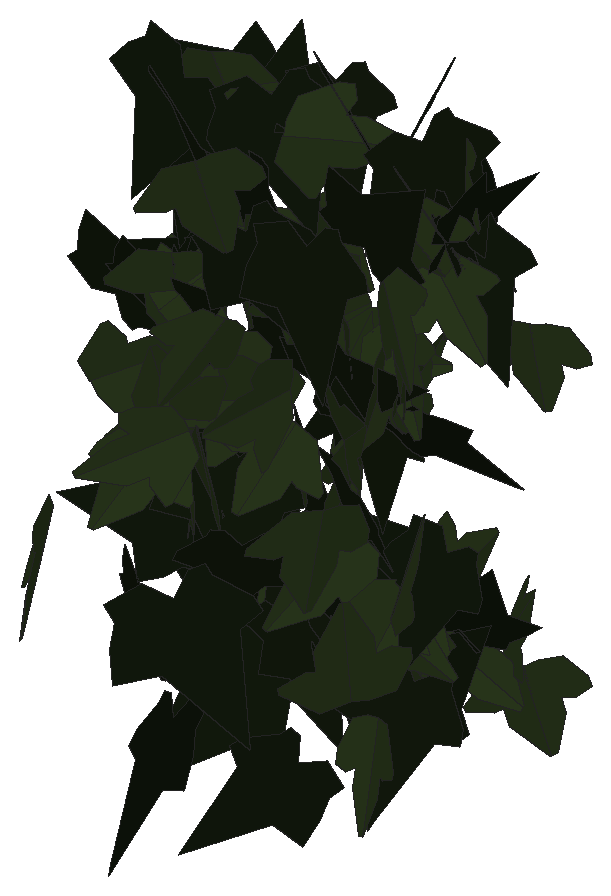
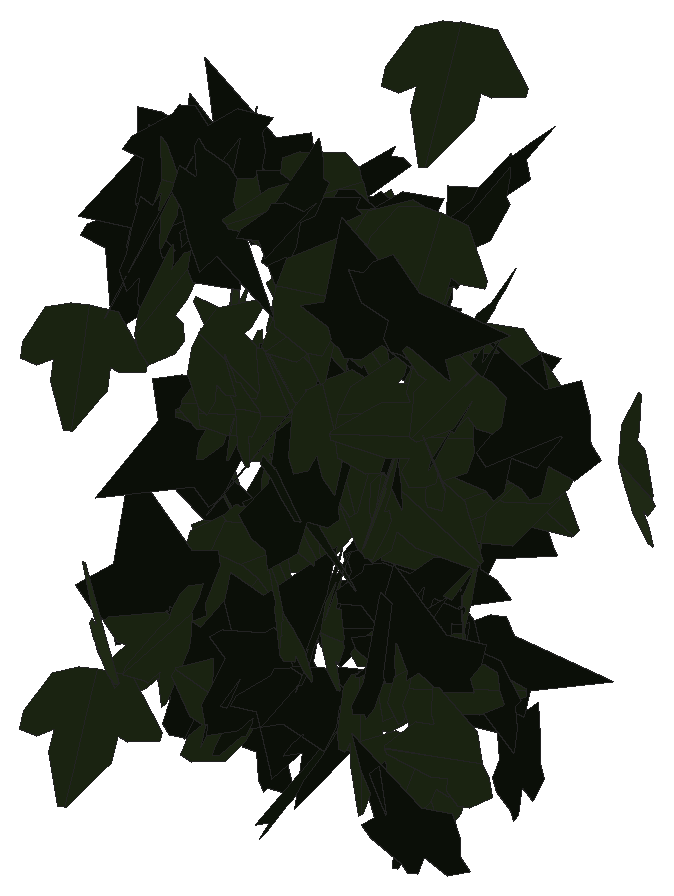
# SketchUp Ruby script. Lengths in inches.
U = 1.inch
M = Sketchup.active_model
def pt(a) = Geom::Point3d.new(a.map { |v| v * U })
def face(e, loops, mat)
  f = e.add_face(loops[0].map { |a| pt(a) })
  loops[1..].each { |l| e.add_face(l.map { |a| pt(a) }).erase! }
  f.material = f.back_material = mat if mat
  f
end
# faces: each face lists its corners as indices into pts; further lists are holes
def faces(e, pts, list, mat = nil) = list.each { |f| face(e, (f[0].is_a?(Array) ? f : [f]).map { |l| l.map { |i| pts[i] } }, mat) }
# xy, xz, yz: faces in a plane at the given z, y or x. An outline is a flat list of corners, or four numbers for a rectangle; further outlines are holes
def ring(l) = l.size == 4 ? [[l[0], l[1]], [l[2], l[1]], [l[2], l[3]], [l[0], l[3]]] : l.each_slice(2).to_a
def flat(e, list, mat, &to3) = list.each { |f| face(e, (f[0].is_a?(Array) ? f : [f]).map { |l| ring(l).map { |u, v| to3.(u, v) } }, mat) }
def xy(e, z, list, mat = nil) = flat(e, list, mat) { |x, y| [x, y, z] }
def xz(e, y, list, mat = nil) = flat(e, list, mat) { |x, z| [x, y, z] }
def yz(e, x, list, mat = nil) = flat(e, list, mat) { |y, z| [x, y, z] }
def lines(e, pts, list) = list.each { |a, b| e.add_line(pt(pts[a]), pt(pts[b])) }
# prism: a flat outline (further loops are holes) pulled along v
def prism(e, loops, v, mat = nil)
  f = face(e, loops, mat); d = Geom::Vector3d.new(v.map { |x| x * U })
  f.pushpull(f.normal.samedirection?(d) ? d.length : -d.length)
end
def box(e, o, s, mat = nil) = prism(e, [[o, [o[0] + s[0], o[1], o[2]], [o[0] + s[0], o[1] + s[1], o[2]], [o[0], o[1] + s[1], o[2]]]], [0, 0, s[2]], mat)
def at(x, y, z, deg = 0) = Geom::Transformation.translation(pt([x, y, z])) * Geom::Transformation.rotation(ORIGIN, Z_AXIS, deg.degrees)
def axes(o, x, y, z) = Geom::Transformation.new([*x, 0, *y, 0, *z, 0, *pt(o).to_a, 1])
def part(name) = M.definitions.add(name)
# library, detail: a bought-in or finely detailed component or shape, given as its bounding box
def library(name, o, s) = part(name).tap { |d| box(d.entities, o, s) }
def detail(e, o, s) = box(e.add_group.entities, o, s)
def put(e, d, t, mat = nil) = e.add_instance(d, t).tap { |i| i.material = mat if mat }
def group(e, t, mat = nil) = e.add_group.tap { |g| g.transformation = t; g.material = mat if mat }.entities
root = M.entities
M.materials.add("efeu1").color = [18, 25, 13]
M.materials.add("efeu2").color = [43, 57, 29]
c1 = part("ivyleaf_10")
p = [[0,0.5,-0.03],[-0.0625,2.02,-0.43],[-0.19,2.01,-0.46],[-0.54,1.05,-0.29],[-0.52,0.625,-0.18],[-0.83,0.76,-0.28],
  [-1.16,0.64,-0.33],[-1.15,0.33,-0.24],[-0.77,-0.39,0.02],[-0.3,-0.51,0.16],[0.04,-0.48,0.23],[-0.02,2.01,-0.4375],
  [-0.06,2.01,-0.43],[0.04,-0.49,0.23],[0.67,-0.49,0.14],[1.38,0.36,-0.2],[1.375,0.51,-0.24],[0.81,0.65,-0.19],
  [0.62,0.59,-0.15],[0.6,1.09,-0.28],[0.5,1.23,-0.31]]
faces(c1.entities,p,[[0,1,2,3,4,5,6,7,8,9,10],[11,12,0,13,14,15,16,17,18,19,20]],"efeu2")
c2 = part("ivyleaf_9")
p = [[1.54,2.16,1.25],[1.36,2.04,1.19],[-0.21,0.99,0.68],[-0.71,1.11,0.82],[-0.85,0.86,0.67],[-0.8,0.17,0.21],
  [-0.9,-0.01,0.1],[-0.67,-0.16,-0.02],[-0.08,-0.08,-0.05],[-0.03,-0.6,-0.4],[0.65,-0.88,-0.66],[0.83,-0.6,-0.49],
  [1.29,-0.42,-0.43],[1.8125,-0.07,-0.26],[1.21,0.44,0.15]]
faces(c2.entities,p,[[0,1,2,3,4,5,6,7,8,9,10,11,12,13,14]],"efeu1")
put(root,c1,axes([537.25,133.6,181.46],[0.57557,0.24818,0.51363],[0.45043,0.25001,-0.62555],[-0.35004,0.72979,0.03962]))
put(root,c1,axes([537.01,133.92,174.57],[0.1954,0.05851,0.86892],[0.85639,0.14889,-0.20261],[-0.15823,0.87809,-0.02355]))
put(root,c2,axes([537.17,131.61,179.2],[-0.21585,-0.03871,0.90493],[0.74592,-0.53531,0.15502],[0.5138,0.76087,0.1551]))
put(root,c2,axes([538.46,134.02,182.43],[-0.26612,0.12962,0.83782],[-0.7365,0.39956,-0.29576],[-0.41988,-0.78301,-0.01223]))
put(root,c2,axes([538.63,131.59,174.97],[-0.37083,-0.27346,-0.68713],[-0.49143,-0.4833,0.45756],[-0.55265,0.61326,0.05419]))
put(root,c2,axes([537.68,133.11,181.74],[0.09063,-0.70819,0.53318],[0.07182,-0.52833,-0.71396],[0.88355,0.11558,0.00334]))
put(root,c2,axes([537.77,133.33,180.37],[-0.06348,-0.47882,0.77083],[0.07599,-0.7728,-0.47379],[0.90425,0.03133,0.09392]))
put(root,c1,axes([538.62,132.86,174.82],[-0.01712,-0.07094,0.79621],[-0.34555,-0.71749,-0.07135],[0.72082,-0.34564,-0.0153]))
put(root,c1,axes([538.375,133.14,183.65],[-0.81606,-0.18859,-0.13277],[0.12874,0.03255,-0.83757],[0.19136,-0.82615,-0.00269]))
put(root,c2,axes([537.98,131.24,172.64],[-0.04193,-0.01194,0.86813],[0.34833,-0.79636,0.00587],[0.79527,0.34817,0.0432]))
put(root,c1,axes([538.08,130.35,178.27],[-0.26014,-0.32007,0.79563],[0.51114,0.60975,0.41242],[-0.68863,0.57351,0.00556]))
put(root,c1,axes([538.09,133.42,179.41],[0.1015,-0.19936,-0.74319],[0.47513,-0.57341,0.21871],[-0.60525,-0.48357,0.04705]))
put(root,c1,axes([537.95,133.3,180.11],[0.02509,-0.0054,0.92465],[0.67,0.63759,-0.01446],[-0.63726,0.67014,0.0212]))
put(root,c2,axes([538.37,131.97,183.875],[-0.15974,-0.84049,0.4832],[-0.04558,-0.48266,-0.85462],[0.96841,-0.16136,0.03948]))
put(root,c2,axes([538.29,133.49,172.17],[-0.40577,0.25126,0.66866],[0.55816,-0.36837,0.47713],[0.44575,0.68998,0.01123]))
put(root,c2,axes([538.6,133.19,175.41],[-0.64239,-0.06086,0.45253],[0.45611,-0.12191,0.63107],[0.02126,0.77626,0.13459]))
put(root,c2,axes([537.97,131.61,179.07],[-0.02434,-0.21976,0.96131],[0.74537,-0.63368,-0.12599],[0.64562,0.7233,0.1817]))
put(root,c2,axes([538.12,132.31,183.25],[0.20488,-0.61087,0.62806],[0.27591,-0.5672,-0.64168],[0.83156,0.3387,0.05817]))
put(root,c1,axes([538.49,134.51,178.64],[-0.32078,0.40567,0.5683],[0.32601,-0.46603,0.51669],[0.61745,0.45681,0.02243]))
put(root,c1,axes([538.86,131.2,180.4],[-0.86672,-0.50452,-0.01723],[0.01642,0.00604,-1.00286],[0.50454,-0.86687,0.00304]))
put(root,c1,axes([538.48,133.28,173.79],[0.66238,0.43416,0.28408],[0.2397,0.15251,-0.79197],[-0.46015,0.7044,-0.00362]))
put(root,c1,axes([538.92,131.05,177.34],[-0.49938,-0.75998,-0.32042],[-0.17716,-0.26699,0.90937],[-0.80551,0.52987,-0.00136]))
put(root,c2,axes([538.4,131.82,175.14],[-0.31705,-0.13686,-0.90242],[0.87432,0.22871,-0.34187],[0.26202,-0.92875,0.04879]))
put(root,c1,axes([538.88,133.23,175.34],[-0.00253,0.18198,-0.75905],[-0.07402,-0.75569,-0.18093],[-0.77704,0.07139,0.01971]))
put(root,c1,axes([538.6,131.88,175.71],[-0.05133,-0.08634,0.89803],[0.72856,-0.53447,-0.00975],[0.53209,0.72349,0.09998]))
put(root,c2,axes([539.05,133.6,181.67],[-0.76145,-0.03775,0.58295],[0.58283,-0.11392,0.75392],[0.03954,0.95219,0.11331]))
put(root,c2,axes([539.24,133.28,175.1],[-0.11503,-0.49954,0.70126],[0.23468,0.66251,0.51043],[-0.82839,0.25706,0.04723]))
put(root,c1,axes([538.77,127.33,176.54],[0.4502,-0.49021,0.75163],[0.50259,-0.55892,-0.66555],[0.74341,0.67472,-0.00523]))
put(root,c1,axes([539.34,129.83,177.33],[0.52573,0.45595,-0.51321],[-0.38248,-0.34225,-0.69588],[-0.57008,0.65011,-0.00641]))
put(root,c1,axes([538.96,132.59,180.57],[-0.49848,0.52672,-0.46065],[0.30608,-0.34447,-0.7251],[-0.62924,-0.58483,0.01221]))
put(root,c1,axes([539.73,132.21,177.46],[-0.15474,-0.11552,-0.93869],[-0.73583,-0.58286,0.19303],[-0.59417,0.7519,0.00542]))
put(root,c1,axes([538.79,132.37,172.22],[-0.48485,-0.00356,0.85233],[0.79903,-0.34323,0.4531],[0.29669,0.91855,0.17261]))
put(root,c1,axes([538.85,131.23,179.86],[0.57569,0.06226,-0.5923],[0.5811,0.12173,0.5776],[0.13046,-0.81696,0.04092]))
put(root,c1,axes([539.87,132.4,178.15],[-0.49317,-0.46191,0.76436],[-0.51842,-0.56293,-0.67467],[0.72722,-0.71455,0.0374]))
put(root,c1,axes([539.53,133.23,183.08],[-0.11115,-0.46317,0.65253],[-0.1139,-0.64293,-0.47576],[0.79206,-0.15745,0.02316]))
put(root,c2,axes([539.49,132.09,172.17],[-0.02978,-0.08491,0.96584],[0.22835,0.9385,0.08955],[-0.94229,0.23012,-0.00882]))
put(root,c1,axes([539.8125,129.71,177.78],[0.22347,0.19537,-0.81594],[-0.65316,-0.48946,-0.29609],[-0.5266,0.69001,0.021]))
put(root,c1,axes([539.5,133.54,180.03],[-0.17061,-0.18924,0.88257],[0.04144,-0.89889,-0.18472],[0.90168,0.00551,0.17548]))
put(root,c1,axes([539.7,131.17,179.37],[-0.25432,-0.64363,0.4639],[-0.16673,-0.43291,-0.69205],[0.77567,-0.30408,0.00335]))
put(root,c1,axes([539.58,133.42,174.54],[0.08376,-0.86743,-0.26606],[-0.0047,0.26677,-0.87123],[0.9073,0.08147,0.02005]))
put(root,c1,axes([539.43,132.36,175.1],[-0.35825,-0.52162,-0.58592],[0.34617,0.4729,-0.63266],[0.70396,-0.498,0.01293]))
put(root,c2,axes([539.59,133,175.16],[-0.27286,-0.58977,0.52273],[-0.16957,-0.49628,-0.64844],[0.76962,-0.31844,0.04246]))
put(root,c1,axes([539.17,132.65,182.875],[-0.52774,-0.18632,-0.83131],[0.80018,0.22724,-0.55891],[0.29241,-0.95809,0.02911]))
put(root,c1,axes([539.71,131.08,176.07],[-0.72596,0.45602,0.20931],[0.17214,-0.11943,0.85725],[0.4713,0.74603,0.00929]))
put(root,c2,axes([540.14,131.39,173.2],[0.12691,0.04204,-0.83107],[-0.80845,0.20536,-0.11307],[0.19711,0.81524,0.07134]))
put(root,c1,axes([540.21,134.25,182.43],[-0.09238,-0.23371,0.79373],[-0.35876,-0.70837,-0.25033],[0.7456,-0.3698,-0.02211]))
put(root,c2,axes([539.68,132,176.25],[-0.41094,-0.81415,-0.4028],[0.23173,0.33351,-0.91051],[0.87829,-0.46893,0.05176]))
put(root,c2,axes([539.77,132.9,183.55],[-0.24033,-0.65657,-0.61162],[0.18134,0.58458,-0.69879],[0.87879,-0.30018,-0.02307]))
put(root,c2,axes([539.5,132.48,181.94],[0.1448,-0.08938,-0.85635],[0.85765,0.09143,0.13548],[0.07581,-0.86368,0.10296]))
put(root,c2,axes([539.86,132.74,179.625],[-0.36791,-0.0118,-0.83624],[0.8363,0.00157,-0.36796],[0.00619,-0.91359,0.01016]))
put(root,c1,axes([540.4,133.27,179.72],[-0.23818,-0.88275,0.12819],[-0.03834,-0.12243,-0.9143],[0.89118,-0.2412,-0.00507]))
put(root,c2,axes([540.8,130.68,175.4375],[0.28727,0.56812,-0.5511],[-0.23412,-0.49905,-0.6365],[-0.75609,0.37038,-0.0123]))
put(root,c1,axes([540.125,132.26,180.33],[-0.4133,-0.01249,0.7715],[0.77066,-0.05002,0.41204],[0.03821,0.87381,0.03462]))
put(root,c2,axes([540.48,133.88,183.67],[-0.19161,-0.63332,-0.39148],[0.12053,0.37252,-0.66164],[0.73473,-0.22628,0.00645]))
put(root,c1,axes([540.54,133.11,175.32],[0.21805,-0.33188,0.65628],[0.45167,-0.47977,-0.39269],[0.58038,0.49806,0.05904]))
put(root,c1,axes([540.47,134.32,176.15],[0.55566,-0.26871,0.55155],[0.49242,-0.24855,-0.61718],[0.36597,0.74241,-0.007]))
put(root,c2,axes([541.24,132.73,174.74],[0.01924,-0.6235,0.67699],[-0.03753,0.67604,0.6237],[-0.9196,-0.04064,-0.01129]))
put(root,c2,axes([541.32,130.35,173.06],[-0.82582,-0.49425,0.21051],[-0.17496,-0.11756,-0.96236],[0.50793,-0.84408,0.01077]))
put(root,c2,axes([540.59,133.68,177.83],[0.8321,-0.20705,-0.28172],[0.28214,-0.03184,0.85674],[-0.20647,-0.87792,0.03537]))
put(root,c2,axes([540.61,133.85,183.52],[0.26471,-0.46113,0.55577],[0.29422,-0.47171,-0.53152],[0.65951,0.39553,0.01405]))
put(root,c2,axes([541.54,133.17,178.01],[-0.6438,0.42685,-0.05787],[0.04681,-0.03413,-0.77245],[-0.4282,-0.6455,0.00257]))
put(root,c1,axes([540.83,133.25,181.35],[-0.54298,0.17,-0.52108],[0.46805,-0.2379,-0.56533],[-0.28524,-0.71398,0.06429]))
put(root,c2,axes([540.85,132.0625,173.3],[0.16419,-0.76771,-0.44035],[-0.03429,0.44201,-0.78339],[0.88438,0.15967,0.05138]))
put(root,c2,axes([540.99,133.0625,174.2],[-0.21892,-0.68621,-0.51465],[0.18221,0.48182,-0.71995],[0.83818,-0.28397,0.02209]))
put(root,c1,axes([541.3,128.88,184.26],[-0.63594,-0.69411,-0.23654],[0.16057,0.17369,-0.94138],[0.71551,-0.65589,0.00103]))
put(root,c2,axes([540.79,130.94,181.87],[-0.24201,-0.24807,-0.89384],[0.64867,0.61509,-0.34634],[0.66311,-0.69223,0.01258]))
put(root,c1,axes([541.7,132.9,179.87],[0.46796,-0.31059,-0.62601],[-0.52266,0.34455,-0.56165],[0.46387,0.70154,-0.0013]))
put(root,c1,axes([540.88,132.55,183.37],[-0.13176,-0.2106,-0.90531],[0.73363,0.53787,-0.2319],[0.57072,-0.74003,0.08909]))
put(root,c2,axes([540.99,133.28,172.49],[0.38826,-0.6627,0.02723],[0.01362,-0.02357,-0.76806],[0.66312,0.3885,-0.00016]))
put(root,c1,axes([541.68,131.87,181.16],[-0.4809,-0.68642,0.26656],[-0.1382,-0.22858,-0.83794],[0.72327,-0.50007,0.01713]))
put(root,c1,axes([542,133.75,179.35],[0.36127,-0.16034,0.68765],[-0.63595,0.26174,0.39514],[-0.30681,-0.73134,-0.00934]))
put(root,c1,axes([541.82,130.58,178.09],[0.76551,0.14579,-0.33747],[-0.33244,-0.05824,-0.77925],[-0.15692,0.83456,0.00457]))
put(root,c2,axes([541.25,133.31,174.53],[-0.11525,-0.26802,-0.87115],[0.55733,0.67406,-0.28111],[0.72118,-0.56375,0.07803]))
put(root,c1,axes([541.68,132.42,179.83],[-0.48453,0.0994,0.79103],[0.68043,-0.43086,0.47093],[0.41549,0.8215,0.15127]))
put(root,c2,axes([542.37,134.25,183.76],[-0.61838,0.56372,-0.46815],[0.34645,-0.31487,-0.83677],[-0.64569,-0.70882,-0.00062]))
put(root,c1,axes([542.16,134.16,180.68],[-0.04353,-0.6242,0.55645],[0.15214,-0.55382,-0.60934],[0.82226,0.06942,0.1422]))
put(root,c1,axes([542.18,132.36,177.26],[0.24453,-0.81839,0.36845],[0.10482,-0.35323,-0.85414],[0.89137,0.26605,-0.00064]))
put(root,c2,axes([542.61,132.25,173.6],[0.50852,-0.35418,0.69409],[-0.54423,0.43175,0.61903],[-0.55769,-0.74427,0.0288]))
put(root,c2,axes([541.61,132.05,178.61],[0.23273,-0.10442,0.87336],[0.76571,-0.4205,-0.25432],[0.43283,0.80006,-0.01968]))
put(root,c1,axes([541.86,132.68,178.86],[-0.03182,-0.00716,0.86582],[0.58194,0.64136,0.02669],[-0.64113,0.58251,-0.01874]))
put(root,c2,axes([542.24,130.8,182.12],[0.04363,-0.95572,-0.15026],[-0.01164,0.14988,-0.95671],[0.96739,0.0449,-0.00473]))
put(root,c2,axes([542.24,132.92,178.1],[0.16935,-0.88776,0.31715],[0.05595,-0.31219,-0.90376],[0.94105,0.17832,-0.00334]))
put(root,c1,axes([542.76,129.25,179.9],[-0.00639,0.02355,-0.9322],[-0.28346,-0.88815,-0.02049],[-0.88837,0.28322,0.01324]))
put(root,c2,axes([543.05,131.84,171.75],[0.20394,-0.26437,0.74015],[-0.38999,0.62985,0.33243],[-0.68237,-0.43899,0.03122]))
put(root,c2,axes([542.21,133.0625,173.49],[0.40173,-0.55209,0.36953],[0.22967,-0.2898,-0.68265],[0.62338,0.46255,0.01337]))
put(root,c2,axes([542.67,126.26,174.32],[-0.19998,0.24155,-0.98303],[0.66953,-0.71998,-0.31312],[-0.75922,-0.69854,-0.01719]))
put(root,c1,axes([542.76,132.86,172.9375],[0.07942,-0.68397,0.61887],[-0.10284,0.61072,0.68816],[-0.91665,-0.12778,-0.02359]))
put(root,c1,axes([542.73,132.61,178.95],[-0.03778,0.39473,-0.77688],[0.08531,-0.7722,-0.3965],[-0.86722,-0.09316,-0.00516]))
put(root,c1,axes([543.2,132.57,178.54],[0.18505,-0.35823,0.70226],[-0.28293,0.64311,0.40261],[-0.73583,-0.33737,0.0218]))
put(root,c2,axes([542.7,126.39,176.8],[-0.16708,-0.64504,-0.79131],[0.27296,0.74442,-0.66445],[0.98374,-0.31611,0.04997]))
put(root,c1,axes([543.34,130.42,176.38],[0.34109,0.49909,-0.76047],[-0.41999,-0.63401,-0.60447],[-0.80686,0.541,-0.00684]))
put(root,c2,axes([542.78,131.43,177],[0.61388,-0.26296,-0.61355],[0.55446,-0.26329,0.6676],[-0.3717,-0.82703,-0.01745]))
put(root,c2,axes([542.86,131.79,182.08],[-0.26774,-0.05716,0.88124],[0.68652,-0.59269,0.17013],[0.55547,0.70497,0.21449]))
put(root,c1,axes([542.91,132.5,179.67],[0.69662,-0.03017,0.52696],[0.52583,-0.03618,-0.6972],[0.04588,0.87274,-0.01069]))
put(root,c1,axes([543.49,133.32,174.54],[0.1466,0.03095,-0.92298],[0.06199,0.9321,0.0411],[0.92142,-0.06763,0.14408]))
put(root,c2,axes([542.91,133.41,173.42],[0.15841,-0.24023,0.87138],[0.51374,-0.70395,-0.28746],[0.7437,0.53745,0.01297]))
put(root,c1,axes([543.16,130.77,178.52],[-0.52089,0.18994,0.66639],[0.62333,-0.2357,0.55442],[0.30266,0.81231,0.00505]))
put(root,c2,axes([543.36,132.89,183.83],[-0.03934,-0.56855,-0.72009],[0.03731,0.71917,-0.56986],[0.91673,-0.05367,-0.0077]))
put(root,c1,axes([543.25,132.36,179.47],[-0.20106,0.00906,0.79456],[0.60938,-0.52423,0.16018],[0.50996,0.63002,0.12185]))
put(root,c1,axes([543.53,134.01,180.6875],[-0.15111,0.2348,0.91607],[0.36885,-0.83959,0.27604],[0.87079,0.39638,0.04205]))
put(root,c2,axes([543.96,128.26,173.01],[-0.03228,-0.00892,-0.90166],[0.04832,-0.90096,0.00718],[-0.90041,-0.04803,0.03271]))
put(root,c1,axes([543.54,132.12,182.59],[-0.79563,-0.16177,-0.49221],[0.47934,0.11255,-0.81181],[0.19666,-0.92878,-0.01265]))
put(root,c2,axes([543.33,132.625,178.01],[0.77101,0.0822,0.23734],[0.2337,0.04598,-0.77512],[-0.09203,0.8054,0.02003]))
put(root,c2,axes([543.76,134.06,181.54],[0.02575,0.05203,0.86048],[-0.27509,-0.81536,0.05753],[0.81698,-0.27619,-0.00775]))
put(root,c1,axes([543.46,133.74,183.2],[-0.26115,0.25279,-0.71399],[0.45343,-0.55277,-0.36156],[-0.6067,-0.52194,0.03711]))
put(root,c2,axes([543.35,132.81,182.61],[0.61023,-0.1825,-0.46421],[0.44353,-0.13705,0.63693],[-0.2282,-0.75438,-0.00341]))
put(root,c2,axes([543.73,133.25,182.72],[0.52641,-0.39496,-0.54441],[-0.39364,0.37964,-0.65605],[0.54536,0.65526,0.05195]))
put(root,c1,axes([543.65,131.65,174.3],[-0.81053,0.0469,-0.42897],[0.42896,-0.01189,-0.81181],[-0.04702,-0.91697,-0.01142]))
put(root,c2,axes([544.04,131.62,173.25],[-0.74039,-0.49075,-0.31249],[0.26361,0.1679,-0.88825],[0.51865,-0.7859,0.00537]))
put(root,c1,axes([544.18,131.08,175.1875],[0.54305,0.56281,-0.43949],[-0.30487,-0.31655,-0.78208],[-0.64572,0.62277,-0.00035]))
put(root,c2,axes([543.72,132.45,172.58],[-0.25632,0.30771,0.8247],[0.54071,-0.62274,0.40041],[0.69458,0.59835,-0.00737]))
put(root,c1,axes([543.77,131.18,174.77],[-0.46672,-0.07216,-0.68645],[0.69021,-0.04209,-0.46485],[0.00558,-0.82902,0.08335]))
put(root,c1,axes([544.29,129.57,174.28],[-0.60506,-0.78668,-0.1797],[-0.10696,-0.14443,0.99244],[-0.79982,0.61443,0.00322]))
put(root,c1,axes([544.06,130.4,172.64],[0.7628,-0.33876,0.22888],[0.20879,-0.09377,-0.83463],[0.3515,0.79085,-0.00093]))
put(root,c2,axes([543.95,133.1875,181.83],[-0.33172,-0.54805,-0.68858],[0.35509,0.58996,-0.64063],[0.80524,-0.48593,-0.00117]))
put(root,c2,axes([544.25,132.46,182.37],[0.19204,0.32882,0.76951],[0.36466,0.67773,-0.38061],[-0.75319,0.41197,0.01193]))
put(root,c1,axes([544.64,128.18,178.33],[-0.4565,-0.86224,0.07932],[-0.02993,-0.0739,-0.97559],[0.86536,-0.45741,0.0081]))
put(root,c1,axes([544.14,132.39,181.44],[0.59441,0.27666,0.48443],[0.44176,0.19886,-0.65562],[-0.34068,0.74057,-0.00492]))
put(root,c1,axes([544.6,130.375,182.06],[-0.25811,0.83548,0.0138],[-0.00594,0.0126,-0.87444],[-0.83558,-0.25817,0.00196]))
put(root,c1,axes([544.34,132.625,173.64],[0.29656,0.48312,0.58567],[0.29973,0.5032,-0.56685],[-0.69755,0.42161,0.00543]))
put(root,c2,axes([544.91,131.5,176.33],[-0.72618,-0.26803,-0.29018],[0.2691,0.10891,-0.77402],[0.28918,-0.77439,-0.00842]))
put(root,c1,axes([544.68,130.57,175.8],[0.5439,-0.68179,-0.08583],[0.05593,-0.06518,0.87216],[-0.68489,-0.54676,0.00305]))
put(root,c2,axes([544.53,132.53,174.27],[0.76338,0.25651,0.13275],[-0.12548,-0.04332,0.80533],[0.26014,-0.77363,-0.00108]))
put(root,c1,axes([545.0625,134,179.9],[-0.78688,-0.31021,-0.01961],[0.01831,0.00701,-0.84582],[0.31029,-0.7871,0.00019]))
put(root,c1,axes([545.1,133.76,172.82],[-0.66583,-0.61868,-0.19706],[0.14551,0.13289,-0.90889],[0.63279,-0.68154,0.00166]))
put(root,c1,axes([544.73,133.77,173.67],[0.39908,-0.51959,-0.47396],[0.305,-0.36317,0.65495],[-0.63371,-0.502,0.01675]))
